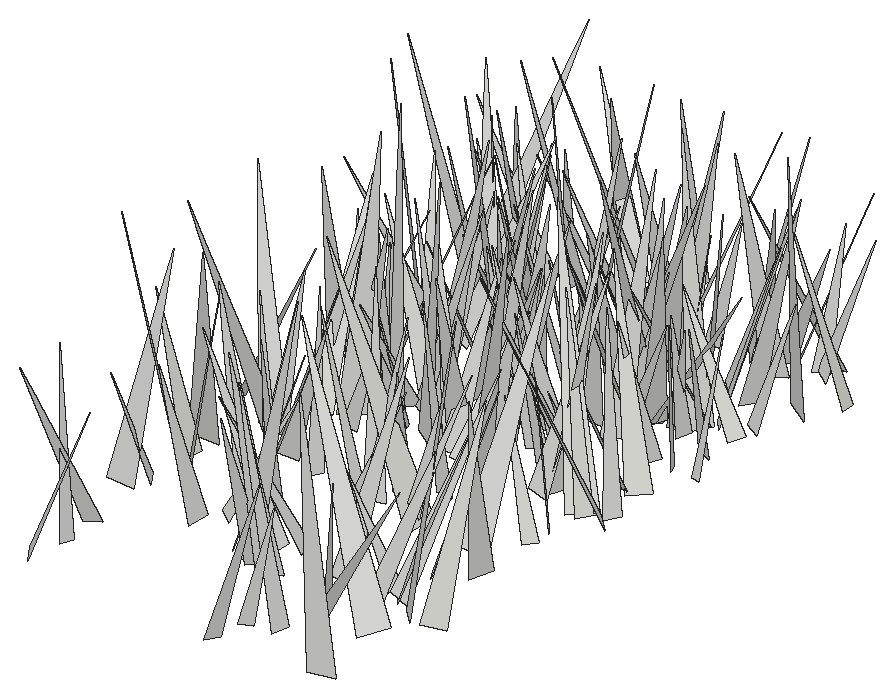
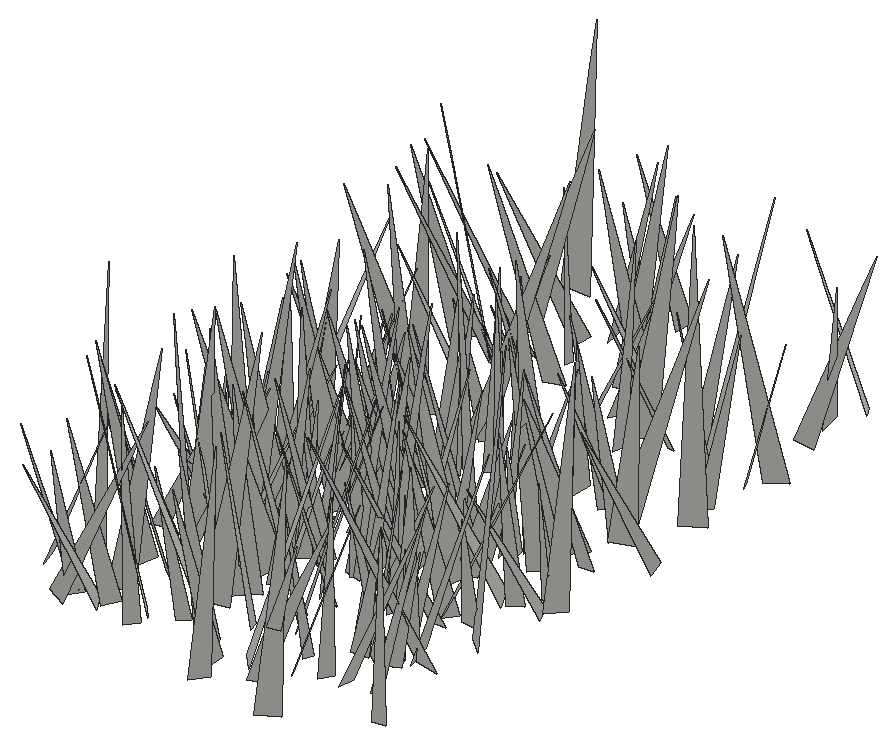
# SketchUp Ruby script. Lengths in inches.
U = 1.inch
M = Sketchup.active_model
def pt(a) = Geom::Point3d.new(a.map { |v| v * U })
def face(e, loops, mat)
  f = e.add_face(loops[0].map { |a| pt(a) })
  loops[1..].each { |l| e.add_face(l.map { |a| pt(a) }).erase! }
  f.material = f.back_material = mat if mat
  f
end
# faces: each face lists its corners as indices into pts; further lists are holes
def faces(e, pts, list, mat = nil) = list.each { |f| face(e, (f[0].is_a?(Array) ? f : [f]).map { |l| l.map { |i| pts[i] } }, mat) }
# xy, xz, yz: faces in a plane at the given z, y or x. An outline is a flat list of corners, or four numbers for a rectangle; further outlines are holes
def ring(l) = l.size == 4 ? [[l[0], l[1]], [l[2], l[1]], [l[2], l[3]], [l[0], l[3]]] : l.each_slice(2).to_a
def flat(e, list, mat, &to3) = list.each { |f| face(e, (f[0].is_a?(Array) ? f : [f]).map { |l| ring(l).map { |u, v| to3.(u, v) } }, mat) }
def xy(e, z, list, mat = nil) = flat(e, list, mat) { |x, y| [x, y, z] }
def xz(e, y, list, mat = nil) = flat(e, list, mat) { |x, z| [x, y, z] }
def yz(e, x, list, mat = nil) = flat(e, list, mat) { |y, z| [x, y, z] }
def lines(e, pts, list) = list.each { |a, b| e.add_line(pt(pts[a]), pt(pts[b])) }
# prism: a flat outline (further loops are holes) pulled along v
def prism(e, loops, v, mat = nil)
  f = face(e, loops, mat); d = Geom::Vector3d.new(v.map { |x| x * U })
  f.pushpull(f.normal.samedirection?(d) ? d.length : -d.length)
end
def box(e, o, s, mat = nil) = prism(e, [[o, [o[0] + s[0], o[1], o[2]], [o[0] + s[0], o[1] + s[1], o[2]], [o[0], o[1] + s[1], o[2]]]], [0, 0, s[2]], mat)
def at(x, y, z, deg = 0) = Geom::Transformation.translation(pt([x, y, z])) * Geom::Transformation.rotation(ORIGIN, Z_AXIS, deg.degrees)
def axes(o, x, y, z) = Geom::Transformation.new([*x, 0, *y, 0, *z, 0, *pt(o).to_a, 1])
def part(name) = M.definitions.add(name)
# library, detail: a bought-in or finely detailed component or shape, given as its bounding box
def library(name, o, s) = part(name).tap { |d| box(d.entities, o, s) }
def detail(e, o, s) = box(e.add_group.entities, o, s)
def put(e, d, t, mat = nil) = e.add_instance(d, t).tap { |i| i.material = mat if mat }
def group(e, t, mat = nil) = e.add_group.tap { |g| g.transformation = t; g.material = mat if mat }.entities
root = M.entities
c1 = part("fur_instance\#9")
p = [[0.8125,0,1.79],[0.67,-0.02,1.48],[0,-0.11,0],[0,0.11,0]]
faces(c1.entities,p,[[0,1,2,3]])
put(root,c1,axes([505.15,195.51,-21.66],[-7.20158,-1.52489,0.67202],[-1.60184,7.15641,-0.92717],[0.45935,1.04894,7.30263]))
put(root,c1,axes([503.36,174.99,-21.66],[-4.62696,1.13691,1.70574],[1.48296,4.76376,0.84751],[1.41525,-1.27471,4.68861]))
put(root,c1,axes([501.49,181.1875,-21.66],[4.45385,0.90104,0.34779],[0.77968,-4.32278,1.21461],[-0.57002,1.12752,4.37874]))
put(root,c1,axes([503.64,166.69,-21.66],[0.77993,-5.26102,0.56712],[-5.12867,-0.89269,-1.22806],[-1.30258,0.36472,5.1748]))
put(root,c1,axes([503.98,164.23,-21.66],[-5.02502,0.15502,0.9974],[-0.08895,4.97687,-1.22169],[1.00545,1.21508,4.87671]))
put(root,c1,axes([504.36,180.21,-21.66],[-3.46559,5.8146,1.30946],[5.95968,3.40104,0.67057],[0.08042,-1.46897,6.73574]))
put(root,c1,axes([503.27,171.86,-21.66],[-3.15969,-2.10838,0.70871],[-1.88389,3.19122,1.09464],[1.18257,-0.54957,3.6374]))
put(root,c1,axes([503.59,187.24,-21.66],[0.89714,3.83975,1.01573],[3.88067,-1.06922,0.61438],[-0.84607,-0.83267,3.89501]))
put(root,c1,axes([502.62,187.7,-21.66],[5.63565,-3.00774,1.4531],[-2.80235,-5.80815,-1.15361],[-1.81792,-0.37081,6.28301]))
put(root,c1,axes([502.48,201.99,-21.66],[-0.50328,-4.91347,1.0032],[-4.85841,0.72759,1.12622],[1.24277,0.85458,4.80907]))
put(root,c1,axes([502.27,170.61,-21.66],[-0.87926,6.56228,2.62812],[6.83144,1.46959,-1.38397],[1.81713,-2.34956,6.47466]))
put(root,c1,axes([503.63,192.86,-21.66],[-5.15951,-5.90719,2.53837],[-5.9684,5.61072,0.92562],[2.3909,1.25844,7.78837]))
put(root,c1,axes([505.16,179.29,-21.66],[-0.75565,-7.24529,1.23648],[-7.25287,0.53359,-1.30585],[-1.19119,1.34729,7.16659]))
put(root,c1,axes([505.07,191.43,-21.66],[-0.56854,4.75375,0.07359],[4.64609,0.5398,1.02436],[-1.0087,-0.19303,4.67676]))
put(root,c1,axes([503.01,188.3,-21.66],[4.04294,1.47662,0.10602],[1.40514,-3.92456,1.07725],[-0.46609,0.97696,4.16717]))
put(root,c1,axes([505.51,197.08,-21.66],[-2.80157,3.07223,0.58027],[3.12461,2.72376,0.66487],[-0.11008,-0.87559,4.10431]))
put(root,c1,axes([504.36,199.87,-21.66],[-1.82022,-4.66244,0.24993],[-4.60062,1.83672,0.75812],[0.79693,-0.04591,4.9474]))
put(root,c1,axes([506.3,199.8125,-21.66],[-5.398,0.07669,0.31538],[0.11355,5.36878,0.63804],[0.30406,-0.64352,5.36071]))
put(root,c1,axes([502.73,176.68,-21.66],[1.80193,-7.44469,0.50754],[-7.36471,-1.69029,1.35351],[1.20089,0.80465,7.53912]))
put(root,c1,axes([506.57,170.74,-21.66],[-6.42891,-4.93695,1.78859],[-5.18873,6.40682,-0.96596],[0.80598,1.86616,8.04806]))
put(root,c1,axes([506.96,191.0625,-21.66],[-5.82237,-2.50943,0.01956],[-2.48564,5.77362,0.82736],[0.34528,-0.75212,6.28591]))
put(root,c1,axes([505.96,177.93,-21.66],[0.1057,3.9764,0.92499],[3.9126,-0.36287,1.11284],[-1.16573,-0.85739,3.81897]))
put(root,c1,axes([506.5,194.79,-21.66],[-2.09458,6.39775,0.76013],[6.40195,1.97698,1.00139],[-0.72385,-1.02792,6.657]))
put(root,c1,axes([503.24,162.12,-21.66],[4.3525,2.53578,0.43229],[2.57081,-4.2585,-0.90411],[0.08934,-0.99816,4.9555]))
put(root,c1,axes([505.54,182.35,-21.66],[-3.21539,5.33291,0.27404],[5.21793,3.20577,-1.16191],[1.13501,0.36996,6.11789]))
put(root,c1,axes([504.93,172.57,-21.66],[4.32331,2.64676,1.47041],[2.57631,-4.56233,0.63737],[-1.59061,-0.19566,5.02892]))
put(root,c1,axes([506.01,195.67,-21.66],[2.91004,3.86675,2.0314],[3.84438,-3.42612,1.0144],[-2.0734,-0.92551,4.73192]))
put(root,c1,axes([504.6,188.47,-21.66],[1.60896,-4.17155,1.4473],[-4.41412,-1.4813,0.63763],[0.1098,1.57772,4.42538]))
put(root,c1,axes([506.41,194.63,-21.66],[-1.858,-4.3991,1.45242],[-4.62148,1.65138,-0.9103],[-0.32175,1.68364,4.68782]))
put(root,c1,axes([504.69,180.07,-21.66],[-2.17172,3.54056,2.13295],[3.72846,2.71807,-0.7156],[1.78427,-1.37037,4.09143]))
put(root,c1,axes([504.21,183.31,-21.66],[1.48764,5.46016,1.29529],[5.56167,-1.25605,-1.09283],[0.74757,-1.52092,5.55267]))
put(root,c1,axes([504.14,196.08,-21.66],[2.50136,7.65725,0.1478],[7.63522,-2.48107,-0.67805],[0.59891,-0.35058,8.02686]))
put(root,c1,axes([507.57,197.16,-21.66],[-1.66438,3.94539,0.96796],[4.04045,1.49913,0.83702],[-0.42169,-1.20819,4.19948]))
put(root,c1,axes([506.88,197.02,-21.66],[-3.29784,-3.61715,1.25797],[-3.53735,3.51322,0.8285],[1.46745,0.33986,4.82422]))
put(root,c1,axes([508.39,187.62,-21.66],[-3.73959,3.61146,1.09906],[3.77498,3.58144,1.07604],[0.00944,-1.53809,5.08619]))
put(root,c1,axes([507.64,184.61,-21.66],[-4.10668,0.43412,1.0008],[0.12519,4.05996,-1.24738],[1.0837,1.17608,3.93666]))
put(root,c1,axes([505.51,188.26,-21.66],[5.65943,2.62486,0.30549],[2.50558,-5.55953,1.3513],[-0.8398,1.10185,6.0904]))
put(root,c1,axes([506.24,178.23,-21.66],[4.19181,1.99584,0.5753],[1.88629,-4.2003,0.82769],[-0.86965,0.50967,4.56832]))
put(root,c1,axes([508.57,184.3,-21.66],[-5.92753,-0.80933,1.51712],[-1.07571,5.99367,-1.00549],[1.34146,1.2301,5.89742]))
put(root,c1,axes([507.69,170.05,-21.66],[-4.50462,1.14541,2.32905],[1.86637,4.67145,1.31236],[1.80364,-1.97324,4.45884]))
put(root,c1,axes([506.71,196.46,-21.66],[0.82444,4.69785,1.50621],[4.90559,-0.61872,-0.75536],[0.52313,-1.60174,4.70945]))
put(root,c1,axes([505.89,184.87,-21.66],[3.45559,-4.90486,0.92565],[-4.98413,-3.32981,0.96246],[0.2699,1.30779,5.9222]))
put(root,c1,axes([507.07,183.29,-21.66],[-5.12716,5.45276,3.67809],[5.84452,5.9162,-0.62364],[3.01704,-2.19425,7.45865]))
put(root,c1,axes([509.77,202.4375,-21.66],[-3.53792,4.34861,0.23075],[4.30519,3.44804,1.02808],[-0.65501,-0.82532,5.51093]))
put(root,c1,axes([506.51,191.38,-21.66],[2.49544,-4.2024,1.5625],[-4.46283,-2.15679,1.32672],[0.42981,2.0042,4.70396]))
put(root,c1,axes([507.45,199.98,-21.66],[4.3427,-1.50818,1.19732],[-1.3579,-4.49272,-0.73402],[-1.36538,-0.32877,4.53816]))
put(root,c1,axes([508.86,184.29,-21.66],[2.99088,7.34321,2.70362],[7.47912,-3.53374,1.32409],[-2.30112,-1.94104,7.81761]))
put(root,c1,axes([506.48,192.32,-21.66],[1.55452,5.85258,0.28483],[5.77094,-1.47817,-1.12324],[1.01494,-0.55917,5.95042]))
put(root,c1,axes([509.05,200.57,-21.66],[-4.05728,-2.523,0.42943],[-2.40041,4.03064,1.00168],[0.88766,-0.63233,4.67158]))
put(root,c1,axes([508.38,195.95,-21.66],[-2.6676,-6.3456,1.58153],[-6.4273,2.85927,0.63121],[1.20736,1.20081,6.85451]))
put(root,c1,axes([508.82,185.79,-21.66],[1.51991,-3.61395,0.26794],[-3.4425,-1.53065,-1.11749],[-1.13207,-0.1975,3.75792]))
put(root,c1,axes([509.875,183.97,-21.66],[-3.12705,-1.8127,0.50032],[-1.87769,2.95706,-1.02213],[-0.10232,1.13341,3.46693]))
put(root,c1,axes([507.27,204.82,-21.66],[4.70982,-4.44224,0.12242],[-4.38661,-4.67586,-0.90827],[-0.71149,-0.57769,6.41023]))
put(root,c1,axes([509.64,193.37,-21.66],[-1.12963,-3.6746,0.26296],[-3.62855,1.06225,-0.74377],[-0.63679,0.46567,3.77168]))
put(root,c1,axes([509.35,177.26,-21.66],[-4.59387,1.36569,1.34916],[1.20913,4.77619,-0.71765],[1.49109,0.33451,4.73854]))
put(root,c1,axes([507.17,177.83,-21.66],[2.31038,-4.41979,0.71264],[-4.3801,-2.06578,1.38834],[0.92579,1.25629,4.79008]))
put(root,c1,axes([507.74,182,-21.66],[1.20072,-3.47995,0.99765],[-3.52529,-0.88496,1.15597],[0.82322,1.28603,3.49507]))
put(root,c1,axes([510.92,185.49,-21.66],[-5.72971,0.10944,0.75393],[-0.02545,5.68949,-1.01935],[0.7614,1.01378,5.63937]))
put(root,c1,axes([511.85,196.5,-21.66],[-7.0839,-2.86843,1.00142],[-2.98784,7.03787,-0.97651],[0.55097,1.28563,7.57997]))
put(root,c1,axes([508.46,188.35,-21.66],[6.64236,-2.17739,2.19825],[-2.53423,-6.81539,0.90685],[-1.77512,1.5823,6.93106]))
put(root,c1,axes([510.375,171.24,-21.66],[-3.35147,5.54659,2.9979],[6.27053,3.28643,0.92965],[0.65767,-3.06906,6.41348]))
put(root,c1,axes([508.99,192.77,-21.66],[4.7247,0.27251,1.48983],[0.66278,-4.76043,-1.23114],[-1.36183,-1.37139,4.56961]))
put(root,c1,axes([511.8,177.63,-21.66],[-4.83845,-0.36416,0.05457],[-0.36621,4.6838,-1.21411],[-0.03844,1.21473,4.69778]))
put(root,c1,axes([511.32,199.49,-21.66],[-0.67131,-4.1889,0.93111],[-4.10147,0.34927,-1.38579],[-1.26165,1.09345,4.00962]))
put(root,c1,axes([510.14,190.03,-21.66],[-2.61623,-5.06997,0.16776],[-4.93297,2.58676,1.24576],[1.18261,-0.42604,5.56752]))
put(root,c1,axes([511.47,201.17,-21.66],[-5.81753,-5.50464,0.89808],[-5.45533,5.88597,0.73893],[1.16061,0.07452,7.97488]))
put(root,c1,axes([511.37,189.89,-21.66],[-4.43723,-6.45792,2.6794],[-6.95056,4.4181,-0.86196],[0.75734,2.71083,7.78786]))
put(root,c1,axes([508.52,171.2,-21.66],[2.58495,3.56171,0.23056],[3.43761,-2.40789,-1.34382],[0.96012,-0.96809,4.1907]))
put(root,c1,axes([510.52,172.72,-21.66],[5.22033,-0.21574,2.13038],[0.1303,-5.5713,-0.88347],[-2.13731,-0.86658,5.14955]))
put(root,c1,axes([509.44,198.91,-21.66],[3.62629,-0.3933,0.08931],[-0.3696,-3.56406,-0.68808],[-0.16141,-0.67481,3.58206]))
put(root,c1,axes([512.69,170.14,-21.66],[-6.22259,1.31552,1.1088],[1.51746,6.15727,1.21077],[0.81078,-1.42761,6.24382]))
put(root,c1,axes([509.49,185.48,-21.66],[3.29943,5.39851,1.49465],[5.593,-3.07886,-1.22601],[0.31023,-1.9081,6.20701]))
put(root,c1,axes([510.64,189.93,-21.66],[5.6278,2.51424,1.57514],[2.22036,-5.80941,1.3399],[-1.96786,0.63554,6.01649]))
put(root,c1,axes([510.85,168.92,-21.66],[4.46685,2.95329,0.59597],[2.75098,-4.43263,1.34675],[-1.2285,0.81223,5.18275]))
put(root,c1,axes([512.74,184.15,-21.66],[-2.01026,5.06538,1.49078],[5.275,1.85579,0.80751],[-0.23431,-1.67916,5.38954]))
put(root,c1,axes([513.25,192.98,-21.66],[-6.49961,-2.89491,2.26898],[-3.37847,6.5202,-1.35892],[1.4542,2.20912,6.98418]))
put(root,c1,axes([513.59,171.16,-21.66],[-4.70083,-1.74871,0.0814],[-1.70109,4.61801,0.97093],[0.41342,-0.88228,4.92068]))
put(root,c1,axes([510.79,188.03,-21.66],[6.83211,0.09479,1.62922],[-0.11306,-6.96812,0.87954],[-1.62805,0.88169,6.77592]))
put(root,c1,axes([511.42,183.45,-21.66],[-3.32783,-6.52848,3.29816],[-6.89122,4.01297,0.99019],[2.45153,2.41834,7.26051]))
put(root,c1,axes([511.66,196.49,-21.66],[6.24718,3.3719,1.68528],[3.2403,-6.4703,0.93425],[-1.92623,0.05148,7.03734]))
put(root,c1,axes([513.35,176.96,-21.66],[-0.65155,5.99766,1.58433],[6.18323,0.49957,0.65163],[-0.49968,-1.63861,5.99765]))
put(root,c1,axes([512.31,203.99,-21.66],[5.42089,-2.3865,1.81758],[-2.19868,-5.71457,-0.94576],[-2.04078,-0.18248,5.84696]))
put(root,c1,axes([512.04,168.57,-21.66],[6.62959,-1.41825,2.66639],[-1.99694,-6.88369,1.30369],[-2.26567,1.91728,6.65307]))
put(root,c1,axes([512.7,168.38,-21.66],[2.86729,-4.50295,0.62999],[-4.43501,-2.93396,-0.78577],[-1.00209,0.10064,5.2802]))
put(root,c1,axes([514.89,190.83,-21.66],[-5.1041,-1.8904,0.52095],[-1.9461,5.06157,-0.70004],[0.24022,0.83889,5.39772]))
put(root,c1,axes([512.82,191.125,-21.66],[-2.64137,-6.46023,1.04071],[-6.35863,2.79897,1.23619],[1.54452,0.47506,6.86901]))
put(root,c1,axes([511.88,193.875,-21.66],[2.7927,4.03544,0.85961],[4.11922,-2.66751,-0.85986],[0.23622,-1.19268,4.83163]))
put(root,c1,axes([512.71,202.31,-21.66],[5.08359,-0.28901,1.82683],[-0.68576,-5.25683,1.07667],[-1.71772,1.24337,4.97667]))
put(root,c1,axes([513.87,187.57,-21.66],[2.18387,-4.44969,1.85832],[-4.59717,-2.53702,-0.67228],[-1.45572,1.33648,4.91091]))
put(root,c1,axes([513.9375,167.92,-21.66],[1.75802,-6.33898,1.96931],[-6.51413,-2.03906,-0.74828],[-1.27556,1.67662,6.53555]))
put(root,c1,axes([511.62,185.67,-21.66],[5.2265,3.38981,1.10604],[3.55749,-5.09026,-1.20993],[-0.2416,-1.62138,6.11091]))
put(root,c1,axes([513.17,183.28,-21.66],[-3.03856,4.16793,1.35783],[3.96538,3.31773,-1.3102],[1.86846,-0.26309,4.98878]))
put(root,c1,axes([512.81,184.6,-21.66],[4.57924,-4.33247,0.58798],[-4.22206,-4.60304,-1.03525],[-1.13589,-0.35667,6.21836]))
put(root,c1,axes([512.49,191,-21.66],[1.67883,-4.20753,0.33675],[-4.18563,-1.61266,0.71764],[0.54516,0.57551,4.47289]))
put(root,c1,axes([513.13,186.83,-21.66],[3.69206,0.52175,1.19179],[0.74035,-3.79133,-0.63373],[-1.0698,-0.8231,3.6745]))
put(root,c1,axes([512.33,189.64,-21.66],[4.00541,-4.88826,1.49079],[-5.10449,-3.91872,0.86522],[-0.24835,1.7057,6.26017]))
put(root,c1,axes([514.19,195.21,-21.66],[-2.66612,-3.28273,0.28859],[-3.19335,2.6653,0.81637],[0.81369,-0.29607,4.14946]))
put(root,c1,axes([512.45,186.86,-21.66],[4.92372,-1.23429,0.65682],[-1.32256,-4.89156,0.72207],[-0.45359,0.86432,5.02445]))
put(root,c1,axes([514.14,191.7,-21.66],[2.11808,6.39246,0.96016],[6.39192,-2.22182,0.69185],[-0.96378,-0.68681,6.6986]))
put(root,c1,axes([516.68,176.42,-21.66],[-8.04315,1.60644,1.39343],[1.83623,7.99603,1.38066],[1.07265,-1.64234,8.08496]))
put(root,c1,axes([515.35,187.875,-21.66],[0.6602,-3.48398,0.63366],[-3.31771,-0.83389,-1.12823],[-1.23791,0.37685,3.36171]))
put(root,c1,axes([512.89,175.52,-21.66],[2.48404,3.35431,0.63876],[3.34518,-2.23213,-1.28736],[0.685,-1.26336,3.97047]))
put(root,c1,axes([513.93,182.8,-21.66],[-0.30009,3.62925,0.24074],[3.53668,0.34756,-0.831],[0.84929,-0.16496,3.54556]))
put(root,c1,axes([513.48,198.2,-21.66],[4.61843,1.91697,0.98697],[2.11588,-4.47821,-1.2031],[-0.41467,-1.49987,4.85358]))
put(root,c1,axes([515.68,179.63,-21.66],[-1.40726,-4.75955,2.034],[-5.17479,1.24906,-0.65748],[-0.10975,2.13481,4.91949]))
put(root,c1,axes([514.25,200.88,-21.66],[4.29417,-2.87763,1.75823],[-3.19183,-4.38696,0.6155],[-1.08829,1.5119,5.13243]))
put(root,c1,axes([515.02,173.66,-21.66],[1.99951,5.4557,0.6063],[5.41529,-2.06607,0.73224],[-0.89823,-0.31139,5.76424]))
put(root,c1,axes([513.7,185.69,-21.66],[1.63751,6.97927,2.94123],[7.53115,-1.18196,-1.38823],[0.80173,-3.15202,7.03309]))
put(root,c1,axes([516.32,186.19,-21.66],[0.21554,-5.31829,2.18174],[-5.56977,-0.73327,-1.23719],[-1.42193,2.0661,5.17688]))
put(root,c1,axes([513.98,178.52,-21.66],[1.58205,-4.94043,0.08132],[-4.90313,-1.55912,0.66773],[0.6114,0.28046,5.1444]))
put(root,c1,axes([514.8,190.68,-21.66],[2.68991,-2.47286,1.2383],[-2.72716,-2.65872,0.6147],[-0.45937,1.30393,3.60178]))
put(root,c1,axes([514.12,186.51,-21.66],[6.01682,-1.89651,1.60783],[-2.22,-5.99358,1.23799],[-1.11958,1.69241,6.18597]))
put(root,c1,axes([515.14,194.11,-21.66],[4.0127,-3.86264,0.72099],[-3.71726,-4.06564,-1.09277],[-1.27351,-0.30356,5.46147]))
put(root,c1,axes([515.76,190.2,-21.66],[-2.72161,-4.19987,1.18368],[-4.18397,2.90781,0.69726],[1.23872,0.59401,4.95579]))
put(root,c1,axes([517.86,163.85,-21.66],[-6.43885,-0.2283,0.73687],[-0.34147,6.39798,-1.00159],[0.69173,1.03328,6.36457]))
put(root,c1,axes([515.45,184.76,-21.66],[5.24089,-0.83273,1.62957],[-1.05437,-5.41429,0.62423],[-1.49573,0.89885,5.2698]))
put(root,c1,axes([515.875,191.23,-21.66],[3.30583,-2.31707,0.74955],[-2.21165,-3.38553,-0.71128],[-1.01942,-0.16893,3.97384]))
put(root,c1,axes([518.68,186.35,-21.66],[-4.50374,-2.5863,0.2222],[-2.55985,4.35118,-1.23954],[-0.43072,1.18335,5.04343]))
put(root,c1,axes([516.45,197.62,-21.66],[2.5513,-6.67742,1.15565],[-6.68995,-2.67869,-0.70836],[-1.08074,0.81812,7.11304]))
put(root,c1,axes([515.64,195.7,-21.66],[2.0151,-5.02328,1.60572],[-5.27188,-1.87389,0.75376],[0.13771,1.76848,5.35965]))
put(root,c1,axes([517.71,184.89,-21.66],[-1.21907,-3.82959,1.50139],[-4.09681,0.98993,-0.80143],[-0.36895,1.66143,3.93822]))
put(root,c1,axes([517.64,186.625,-21.66],[-5.01187,1.13995,1.85475],[1.60842,5.07616,1.22637],[1.46717,-1.67079,4.99142]))
put(root,c1,axes([515.74,161.09,-21.66],[4.66394,-1.20705,1.00362],[-1.36601,-4.67089,0.73033],[-0.77347,0.97077,4.76192]))
put(root,c1,axes([516.17,163.22,-21.66],[2.59266,-2.6088,0.97622],[-2.78019,-2.50569,0.68761],[-0.17141,1.18171,3.61316]))
put(root,c1,axes([516.2,176.18,-21.66],[-1.839,3.01934,1.93742],[3.07994,2.44517,-0.88715],[1.83955,-1.07548,3.42218]))
put(root,c1,axes([518.76,193.06,-21.66],[-2.91318,-3.12111,0.33199],[-3.12229,2.8354,-0.74159],[-0.32068,0.74655,4.20452]))
put(root,c1,axes([515.82,182.25,-21.66],[7.89082,-0.9052,1.78608],[-0.78265,-8.07818,-0.63641],[-1.84308,-0.44515,7.91703]))
put(root,c1,axes([514.91,199.79,-21.66],[6.15209,3.35933,0.33959],[3.37614,-6.1107,-0.71393],[0.04606,-0.78923,6.97306]))
put(root,c1,axes([516.6,199.85,-21.66],[-0.37702,3.57753,2.02822],[3.88687,0.97529,-0.99777],[1.34335,-1.81786,3.4562]))
put(root,c1,axes([516.71,190.01,-21.66],[1.30695,-5.86281,0.96642],[-5.89292,-1.15208,0.98022],[0.76158,1.14664,5.9262]))
put(root,c1,axes([519.8125,185.18,-21.66],[-5.72076,-3.26575,0.35826],[-3.1922,5.6955,0.94426],[0.77675,-0.64548,6.51924]))
put(root,c1,axes([516.2,196.36,-21.66],[4.17782,-5.39394,0.17375],[-5.37681,-4.14138,0.71959],[0.46328,0.57738,6.78461]))
put(root,c1,axes([517.2,169.62,-21.66],[0.34617,6.42334,1.62872],[6.51894,-0.03728,-1.2385],[1.18972,-1.66468,6.31231]))
put(root,c1,axes([521.65,166.58,-21.66],[-7.18183,4.15456,0.03319],[4.14203,7.15453,0.70461],[-0.3242,-0.62648,8.26695]))
put(root,c1,axes([518.01,193.27,-21.66],[-1.4202,-8.16889,0.91065],[-8.13373,1.52988,1.03868],[1.18423,0.71114,8.22611]))
put(root,c1,axes([517.14,192.14,-21.66],[6.46627,-2.11143,1.67342],[-2.36842,-6.52888,0.91405],[-1.28416,1.40953,6.74057]))
put(root,c1,axes([516.28,193.18,-21.66],[6.91635,-1.96319,0.7746],[-2.05636,-6.86586,0.95992],[-0.47486,1.1384,7.12521]))
put(root,c1,axes([518.89,190.57,-21.66],[-2.89154,-5.8907,0.51675],[-5.81601,2.937,0.93617],[1.06836,0.04534,6.49499]))
put(root,c1,axes([518.68,189.48,-21.66],[5.55139,-3.03279,3.66915],[-4.09539,-5.91606,1.30628],[-2.42657,3.04644,6.18946]))
put(root,c1,axes([519.67,170.73,-21.66],[-3.46593,0.7925,0.89611],[1.04093,3.35143,1.06213],[0.58952,-1.25841,3.39303]))
put(root,c1,axes([517.93,167.55,-21.66],[4.34491,0.59069,1.09524],[0.90101,-4.23706,-1.28924],[-0.85828,-1.45776,4.19106]))
put(root,c1,axes([517.78,191.55,-21.66],[-0.77592,-4.15559,2.31409],[-4.39268,1.52537,1.26634],[1.82437,1.90534,4.03328]))
put(root,c1,axes([519.03,184.49,-21.66],[-3.21117,5.73542,2.2751],[5.803,3.67883,-1.08356],[2.09673,-1.39782,6.48325]))
put(root,c1,axes([521.38,192.75,-21.66],[-7.28379,2.71503,1.56111],[2.64145,7.44897,-0.63058],[1.68261,0.05921,7.74773]))
put(root,c1,axes([518.4,201.75,-21.66],[5.40312,-1.02873,0.51523],[-0.87968,-5.28821,-1.33359],[-0.74156,-1.2223,5.33606]))
put(root,c1,axes([521.29,193.38,-21.66],[-1.6318,-4.41068,0.10105],[-4.3461,1.58854,-0.8456],[-0.75876,0.38671,4.62621]))
put(root,c1,axes([522.17,182.5,-21.66],[-4.81407,6.51041,0.79127],[6.55623,4.75265,0.78417],[-0.16528,-1.10168,8.05889]))
put(root,c1,axes([518.7,190.42,-21.66],[3.23817,-2.36152,0.30304],[-2.37388,-3.16317,0.7165],[0.18248,0.75624,3.94324]))
put(root,c1,axes([519.22,182.62,-21.66],[1.31333,6.20143,0.89],[6.24264,-1.21867,-0.72041],[0.52849,-1.01577,6.2979]))
put(root,c1,axes([518.49,200.4,-21.66],[5.36031,4.39922,1.5205],[4.6383,-5.24227,-1.18439],[-0.38885,-1.88772,6.83252]))
put(root,c1,axes([519.23,193.91,-21.66],[4.62058,2.87983,1.50344],[3.15499,-4.60106,-0.88304],[-0.77446,-1.56215,5.37246]))
put(root,c1,axes([520.99,199.33,-21.66],[1.6386,-6.2759,2.07036],[-6.47654,-1.94928,-0.78297],[-1.31443,1.78093,6.43885]))
put(root,c1,axes([522.33,185.64,-21.66],[-2.45002,-3.17903,0.27674],[-3.09062,2.27713,-1.20338],[-0.79426,0.94543,3.82893]))
put(root,c1,axes([519.83,183.47,-21.66],[5.84499,-0.86217,1.83487],[-1.09003,-6.05756,0.62599],[-1.70936,0.91471,5.87498]))
put(root,c1,axes([522.49,182.36,-21.66],[-5.52094,1.92393,0.48296],[1.85996,5.5174,-0.71721],[0.68943,0.52184,5.80241]))
put(root,c1,axes([522.07,178.48,-21.66],[-2.23276,3.13779,0.67741],[3.20125,2.1153,0.75324],[-0.23799,-0.9847,3.77672]))
put(root,c1,axes([520.26,172.91,-21.66],[4.1336,3.03674,0.5342],[2.87698,-4.11997,1.15876],[-1.10914,0.6308,4.99657]))
put(root,c1,axes([520.33,176.05,-21.66],[-1.86477,7.56726,1.18834],[7.49142,2.05683,-1.34204],[1.5982,-0.81177,7.67722]))
put(root,c1,axes([519.27,191.71,-21.66],[6.44633,-3.37101,0.63256],[-3.2949,-6.46051,-0.8512],[-0.95262,-0.46602,7.22457]))
put(root,c1,axes([518.8,165.45,-21.66],[4.72114,-1.50275,0.05764],[-1.46013,-4.53503,1.361],[0.36002,1.31378,4.76394]))
put(root,c1,axes([519.35,191.93,-21.66],[4.38555,-0.36882,0.03632],[-0.36139,-4.16033,1.38975],[0.08213,1.3878,4.17584]))
put(root,c1,axes([522,180.05,-21.66],[-3.20539,-1.99252,1.2784],[-2.28309,3.17085,-0.78241],[0.62603,1.36182,3.69222]))
put(root,c1,axes([523.08,201.92,-21.66],[-1.88046,-5.21634,0.33238],[-5.10911,1.75978,-1.28722],[-1.10347,0.74146,5.39346]))
put(root,c1,axes([521.6,188.73,-21.66],[3.25434,-3.10316,1.28908],[-2.93626,-3.49873,-1.00964],[-1.63392,0.10675,4.38189]))
put(root,c1,axes([520.37,194.62,-21.66],[5.81902,2.09502,1.94943],[2.48849,-5.88572,-1.1028],[-1.4131,-1.7377,6.08555]))
put(root,c1,axes([521.18,191.82,-21.66],[3.43553,-2.13589,0.95207],[-2.02418,-3.56342,-0.68999],[-1.17096,-0.10667,3.98608]))
put(root,c1,axes([523.21,185.74,-21.66],[-3.60307,5.2202,0.86904],[5.28801,3.51043,0.83765],[-0.20649,-1.18922,6.28736]))
put(root,c1,axes([520.47,192.05,-21.66],[1.50872,-3.69838,0.31644],[-3.67115,-1.43625,0.71715],[0.54852,0.55997,3.92937]))
put(root,c1,axes([522.29,161.59,-21.66],[0.36283,-7.33481,3.26148],[-7.98321,-0.67122,-0.62142],[-0.83968,3.21222,7.31744]))
put(root,c1,axes([523.51,193.11,-21.66],[-3.19624,2.75407,0.40141],[2.73336,2.9911,1.24258],[-0.52417,-1.19599,4.03198]))
put(root,c1,axes([520.2,167.96,-21.66],[2.81698,6.47491,0.35167],[6.46114,-2.77024,-0.75032],[0.54938,-0.62035,7.02117]))
put(root,c1,axes([519.98,196.83,-21.66],[4.42305,4.26534,0.99754],[4.37397,-4.22348,-1.33498],[0.23791,-1.64944,5.99786]))
put(root,c1,axes([520.53,170,-21.66],[1.99959,6.47326,0.24716],[6.43471,-1.95494,-0.85747],[0.74746,-0.48749,6.72058]))
put(root,c1,axes([521.05,201.09,-21.66],[4.24517,2.47398,0.29086],[2.34061,-4.15824,1.20716],[-0.85248,0.90284,4.76286]))
put(root,c1,axes([521.94,168.92,-21.66],[5.36611,5.59511,2.05394],[5.5109,-5.71038,1.15783],[-2.27022,-0.63666,7.66549]))
put(root,c1,axes([520.3,170.1875,-21.66],[4.29759,3.17988,0.45483],[3.21134,-4.23507,-0.73441],[0.07624,-0.86047,5.29543]))
put(root,c1,axes([523.57,182.4,-21.66],[-4.47092,-4.93614,0.16266],[-4.90041,4.46105,0.68268],[0.61475,-0.33851,6.62484]))
put(root,c1,axes([522.89,188.79,-21.66],[-3.3024,-1.44134,1.34219],[-1.74105,3.36144,-0.674],[0.92071,1.18661,3.53964]))
put(root,c1,axes([520.51,200.73,-21.66],[3.4493,-3.36014,0.02886],[-3.29462,-3.37365,0.97621],[0.66096,0.719,4.71542]))
put(root,c1,axes([523.67,183,-21.66],[-5.20641,1.3754,0.94823],[1.21962,5.25029,-0.91901],[1.14166,0.66356,5.30602]))
put(root,c1,axes([521.85,193.72,-21.66],[3.70568,3.40586,0.49894],[3.35111,-3.73706,0.62078],[-0.78668,0.12425,4.99466]))
put(root,c1,axes([522.52,201.08,-21.66],[-2.57998,2.99071,1.64125],[3.02202,2.95835,-0.64026],[1.58287,-0.77341,3.89753]))
put(root,c1,axes([521.78,196.43,-21.66],[5.79665,-1.91222,1.6292],[-2.17494,-5.87047,0.84811],[-1.25719,1.33905,6.04471]))
put(root,c1,axes([522.19,174.47,-21.66],[5.38586,-3.00561,1.16634],[-2.8404,-5.49795,-1.05176],[-1.52519,-0.37466,6.07741]))
put(root,c1,axes([523.14,190.96,-21.66],[-1.38247,-3.90181,0.99129],[-3.91317,1.54858,0.63797],[0.94545,0.70412,4.09003]))
put(root,c1,axes([525.82,199.08,-21.66],[-5.12979,-1.0122,0.11272],[-1.018,5.07872,-0.72273],[-0.03042,0.73083,5.17851]))
put(root,c1,axes([524.41,188.67,-21.66],[1.50713,3.43781,0.3216],[3.3001,-1.53741,0.96906],[-1.01552,0.10596,3.62641]))
put(root,c1,axes([523.62,168.81,-21.66],[-3.09006,5.24053,1.65653],[5.13422,3.43055,-1.27548],[1.9614,-0.72379,5.94851]))
put(root,c1,axes([522.84,200.74,-21.66],[2.35379,3.88662,0.95748],[3.9563,-2.09005,-1.24191],[0.60851,-1.44527,4.3708]))
put(root,c1,axes([524.15,197.17,-21.66],[3.79237,5.90894,3.79832],[6.9076,-3.92109,-0.79686],[-1.27587,-3.6653,6.97586]))
put(root,c1,axes([523.5,194.375,-21.66],[1.6531,3.56586,0.9383],[3.65871,-1.45863,-0.90264],[0.45784,-1.21883,3.82535]))
